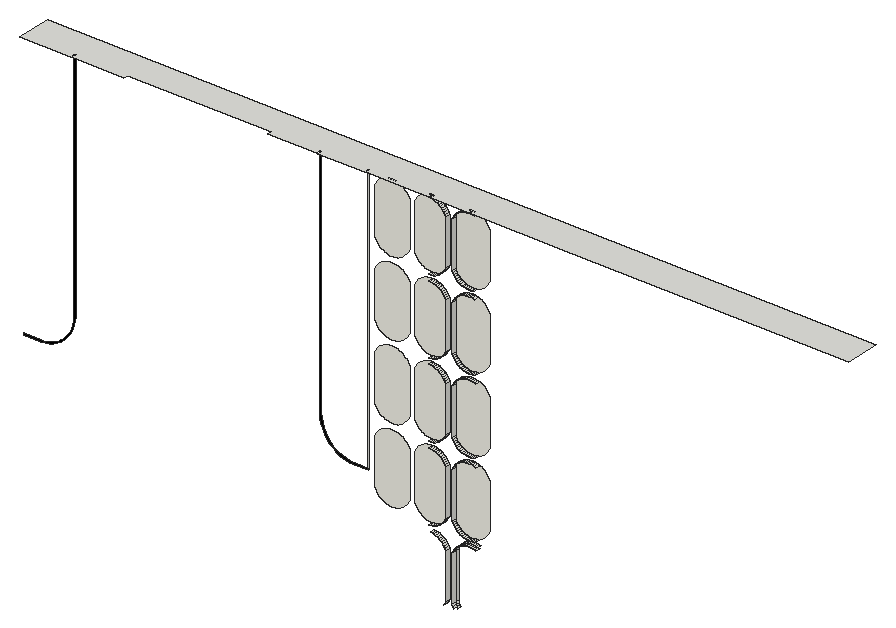
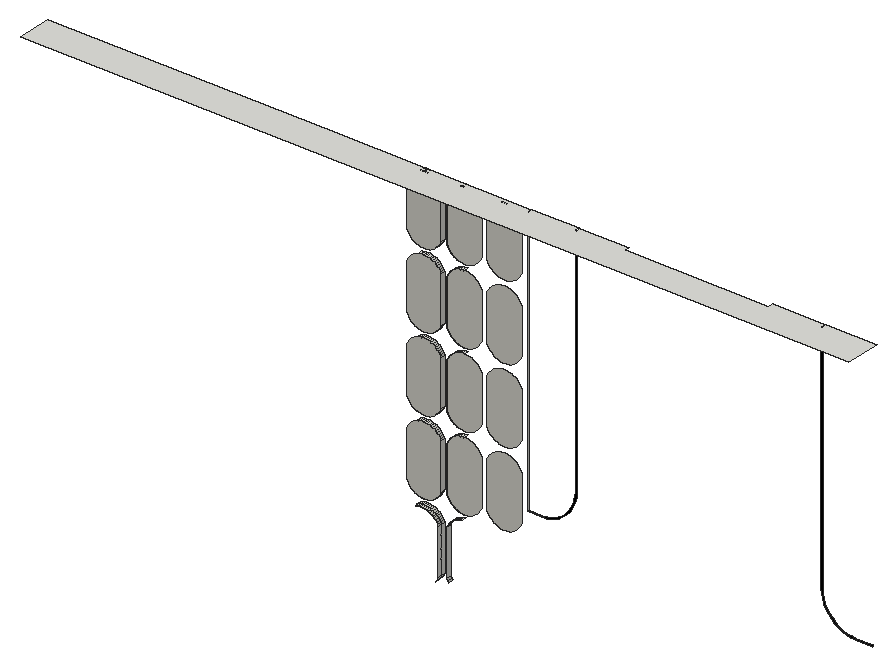
# SketchUp Ruby script. Lengths in inches.
U = 1.inch
M = Sketchup.active_model
def pt(a) = Geom::Point3d.new(a.map { |v| v * U })
def face(e, loops, mat)
  f = e.add_face(loops[0].map { |a| pt(a) })
  loops[1..].each { |l| e.add_face(l.map { |a| pt(a) }).erase! }
  f.material = f.back_material = mat if mat
  f
end
# faces: each face lists its corners as indices into pts; further lists are holes
def faces(e, pts, list, mat = nil) = list.each { |f| face(e, (f[0].is_a?(Array) ? f : [f]).map { |l| l.map { |i| pts[i] } }, mat) }
# xy, xz, yz: faces in a plane at the given z, y or x. An outline is a flat list of corners, or four numbers for a rectangle; further outlines are holes
def ring(l) = l.size == 4 ? [[l[0], l[1]], [l[2], l[1]], [l[2], l[3]], [l[0], l[3]]] : l.each_slice(2).to_a
def flat(e, list, mat, &to3) = list.each { |f| face(e, (f[0].is_a?(Array) ? f : [f]).map { |l| ring(l).map { |u, v| to3.(u, v) } }, mat) }
def xy(e, z, list, mat = nil) = flat(e, list, mat) { |x, y| [x, y, z] }
def xz(e, y, list, mat = nil) = flat(e, list, mat) { |x, z| [x, y, z] }
def yz(e, x, list, mat = nil) = flat(e, list, mat) { |y, z| [x, y, z] }
def lines(e, pts, list) = list.each { |a, b| e.add_line(pt(pts[a]), pt(pts[b])) }
# prism: a flat outline (further loops are holes) pulled along v
def prism(e, loops, v, mat = nil)
  f = face(e, loops, mat); d = Geom::Vector3d.new(v.map { |x| x * U })
  f.pushpull(f.normal.samedirection?(d) ? d.length : -d.length)
end
def box(e, o, s, mat = nil) = prism(e, [[o, [o[0] + s[0], o[1], o[2]], [o[0] + s[0], o[1] + s[1], o[2]], [o[0], o[1] + s[1], o[2]]]], [0, 0, s[2]], mat)
def at(x, y, z, deg = 0) = Geom::Transformation.translation(pt([x, y, z])) * Geom::Transformation.rotation(ORIGIN, Z_AXIS, deg.degrees)
def axes(o, x, y, z) = Geom::Transformation.new([*x, 0, *y, 0, *z, 0, *pt(o).to_a, 1])
def part(name) = M.definitions.add(name)
# library, detail: a bought-in or finely detailed component or shape, given as its bounding box
def library(name, o, s) = part(name).tap { |d| box(d.entities, o, s) }
def detail(e, o, s) = box(e.add_group.entities, o, s)
def put(e, d, t, mat = nil) = e.add_instance(d, t).tap { |i| i.material = mat if mat }
def group(e, t, mat = nil) = e.add_group.tap { |g| g.transformation = t; g.material = mat if mat }.entities
root = M.entities
M.materials.add("Tafisa-Gardenia-or-Gardenia-PM775-4K").color = [246, 245, 235]
M.materials.add("[Color M09]").color = [0, 0, 0]
xy(root,114,[[4.5,138,13.26,138,13.26,138.71,13.5,138.71,13.5,138,22.5,138,22.5,138.79,47.5,138.79,47.5,138,56,138,56,138.71,56.24,138.71,56.24,138,64.38,138,64.38,138.71,64.5,138.71,64.5,138,100.5,138,100.5,138.71,100.62,138.71,100.62,138,148.5,138,148.5,144,4.5,144]])
xz(root,138.71,[[64.38,67.55,64.5,114]])
xz(root,138.71,[[4.5,67.3125,7.5,67.3125,8.28,67.36,9.05,67.52,9.8,67.77,10.5,68.12,11.15,68.55,11.74,69.07,12.26,69.66,12.7,70.3125,13.04,71.02,13.3,71.76,13.45,72.53,13.5,73.3125,13.5,114,13.26,114,13.26,73.3125,13.21,72.56,13.07,71.82,12.83,71.11,12.49,70.43,12.07,69.8,11.58,69.24,11.01,68.74,10.38,68.32,9.71,67.99,8.99,67.75,8.25,67.6,7.5,67.55,4.5,67.55],[62,67.3125,64.5,67.3125,64.5,67.55,62,67.55,61.25,67.6,60.51,67.75,59.79,67.99,59.12,68.32,58.49,68.74,57.92,69.24,57.43,69.8,57.01,70.43,56.67,71.11,56.43,71.82,56.29,72.56,56.24,73.3125,56.24,114,56,114,56,73.3125,56.05,72.53,56.2,71.76,56.46,71.02,56.8,70.3125,57.24,69.66,57.76,69.07,58.35,68.55,59,68.12,59.7,67.77,60.45,67.52,61.22,67.36]],"[Color M09]")
xz(root,138.79,[[68.5,63,68.82,63.02,69.13,63.0625,69.44,63.14,69.74,63.25,70.03,63.38,70.3,63.55,70.56,63.74,70.79,63.95,71.01,64.18,71.2,64.44,71.36,64.71,71.5,65,71.5,73,71.36,73.29,71.2,73.56,71.01,73.82,70.79,74.05,70.56,74.26,70.3,74.45,70.03,74.62,69.74,74.75,69.44,74.86,69.13,74.9375,68.82,74.98,68.5,75,68.18,74.98,67.87,74.9375,67.56,74.86,67.26,74.75,66.97,74.62,66.7,74.45,66.44,74.26,66.21,74.05,65.99,73.82,65.8,73.56,65.64,73.29,65.5,73,65.5,65,65.64,64.71,65.8,64.44,65.99,64.18,66.21,63.95,66.44,63.74,66.7,63.55,66.97,63.38,67.26,63.25,67.56,63.14,67.87,63.0625,68.18,63.02],[75.5,63,75.82,63.02,76.13,63.0625,76.44,63.14,76.74,63.25,77.03,63.38,77.3,63.55,77.56,63.74,77.79,63.95,78.01,64.18,78.2,64.44,78.36,64.71,78.5,65,78.5,73,78.36,73.29,78.2,73.56,78.01,73.82,77.79,74.05,77.56,74.26,77.3,74.45,77.03,74.62,76.74,74.75,76.44,74.86,76.13,74.9375,75.82,74.98,75.5,75,75.18,74.98,74.87,74.9375,74.56,74.86,74.26,74.75,73.97,74.62,73.7,74.45,73.44,74.26,73.21,74.05,72.99,73.82,72.8,73.56,72.64,73.29,72.5,73,72.5,65,72.64,64.71,72.8,64.44,72.99,64.18,73.21,63.95,73.44,63.74,73.7,63.55,73.97,63.38,74.26,63.25,74.56,63.14,74.87,63.0625,75.18,63.02],[82.5,63,82.82,63.02,83.13,63.0625,83.44,63.14,83.74,63.25,84.03,63.38,84.3,63.55,84.56,63.74,84.79,63.95,85.01,64.18,85.2,64.44,85.36,64.71,85.5,65,85.5,73,85.36,73.29,85.2,73.56,85.01,73.82,84.79,74.05,84.56,74.26,84.3,74.45,84.03,74.62,83.74,74.75,83.44,74.86,83.13,74.9375,82.82,74.98,82.5,75,82.18,74.98,81.87,74.9375,81.56,74.86,81.26,74.75,80.97,74.62,80.7,74.45,80.44,74.26,80.21,74.05,79.99,73.82,79.8,73.56,79.64,73.29,79.5,73,79.5,65,79.64,64.71,79.8,64.44,79.99,64.18,80.21,63.95,80.44,63.74,80.7,63.55,80.97,63.38,81.26,63.25,81.56,63.14,81.87,63.0625,82.18,63.02],[68.5,76,68.82,76.02,69.13,76.0625,69.44,76.14,69.74,76.25,70.03,76.38,70.3,76.55,70.56,76.74,70.79,76.95,71.01,77.18,71.2,77.44,71.36,77.71,71.5,78,71.5,86,71.36,86.29,71.2,86.56,71.01,86.82,70.79,87.05,70.56,87.26,70.3,87.45,70.03,87.62,69.74,87.75,69.44,87.86,69.13,87.9375,68.82,87.98,68.5,88,68.18,87.98,67.87,87.9375,67.56,87.86,67.26,87.75,66.97,87.62,66.7,87.45,66.44,87.26,66.21,87.05,65.99,86.82,65.8,86.56,65.64,86.29,65.5,86,65.5,78,65.64,77.71,65.8,77.44,65.99,77.18,66.21,76.95,66.44,76.74,66.7,76.55,66.97,76.38,67.26,76.25,67.56,76.14,67.87,76.0625,68.18,76.02],[75.5,76,75.82,76.02,76.13,76.0625,76.44,76.14,76.74,76.25,77.03,76.38,77.3,76.55,77.56,76.74,77.79,76.95,78.01,77.18,78.2,77.44,78.36,77.71,78.5,78,78.5,86,78.36,86.29,78.2,86.56,78.01,86.82,77.79,87.05,77.56,87.26,77.3,87.45,77.03,87.62,76.74,87.75,76.44,87.86,76.13,87.9375,75.82,87.98,75.5,88,75.18,87.98,74.87,87.9375,74.56,87.86,74.26,87.75,73.97,87.62,73.7,87.45,73.44,87.26,73.21,87.05,72.99,86.82,72.8,86.56,72.64,86.29,72.5,86,72.5,78,72.64,77.71,72.8,77.44,72.99,77.18,73.21,76.95,73.44,76.74,73.7,76.55,73.97,76.38,74.26,76.25,74.56,76.14,74.87,76.0625,75.18,76.02],
  [82.5,76,82.82,76.02,83.13,76.0625,83.44,76.14,83.74,76.25,84.03,76.38,84.3,76.55,84.56,76.74,84.79,76.95,85.01,77.18,85.2,77.44,85.36,77.71,85.5,78,85.5,86,85.36,86.29,85.2,86.56,85.01,86.82,84.79,87.05,84.56,87.26,84.3,87.45,84.03,87.62,83.74,87.75,83.44,87.86,83.13,87.9375,82.82,87.98,82.5,88,82.18,87.98,81.87,87.9375,81.56,87.86,81.26,87.75,80.97,87.62,80.7,87.45,80.44,87.26,80.21,87.05,79.99,86.82,79.8,86.56,79.64,86.29,79.5,86,79.5,78,79.64,77.71,79.8,77.44,79.99,77.18,80.21,76.95,80.44,76.74,80.7,76.55,80.97,76.38,81.26,76.25,81.56,76.14,81.87,76.0625,82.18,76.02],[68.5,89,68.82,89.02,69.13,89.0625,69.44,89.14,69.74,89.25,70.03,89.38,70.3,89.55,70.56,89.74,70.79,89.95,71.01,90.18,71.2,90.44,71.36,90.71,71.5,91,71.5,99,71.36,99.29,71.2,99.56,71.01,99.82,70.79,100.05,70.56,100.26,70.3,100.45,70.03,100.62,69.74,100.75,69.44,100.86,69.13,100.9375,68.82,100.98,68.5,101,68.18,100.98,67.87,100.9375,67.56,100.86,67.26,100.75,66.97,100.62,66.7,100.45,66.44,100.26,66.21,100.05,65.99,99.82,65.8,99.56,65.64,99.29,65.5,99,65.5,91,65.64,90.71,65.8,90.44,65.99,90.18,66.21,89.95,66.44,89.74,66.7,89.55,66.97,89.38,67.26,89.25,67.56,89.14,67.87,89.0625,68.18,89.02],[75.5,89,75.82,89.02,76.13,89.0625,76.44,89.14,76.74,89.25,77.03,89.38,77.3,89.55,77.56,89.74,77.79,89.95,78.01,90.18,78.2,90.44,78.36,90.71,78.5,91,78.5,99,78.36,99.29,78.2,99.56,78.01,99.82,77.79,100.05,77.56,100.26,77.3,100.45,77.03,100.62,76.74,100.75,76.44,100.86,76.13,100.9375,75.82,100.98,75.5,101,75.18,100.98,74.87,100.9375,74.56,100.86,74.26,100.75,73.97,100.62,73.7,100.45,73.44,100.26,73.21,100.05,72.99,99.82,72.8,99.56,72.64,99.29,72.5,99,72.5,91,72.64,90.71,72.8,90.44,72.99,90.18,73.21,89.95,73.44,89.74,73.7,89.55,73.97,89.38,74.26,89.25,74.56,89.14,74.87,89.0625,75.18,89.02],[82.5,89,82.82,89.02,83.13,89.0625,83.44,89.14,83.74,89.25,84.03,89.38,84.3,89.55,84.56,89.74,84.79,89.95,85.01,90.18,85.2,90.44,85.36,90.71,85.5,91,85.5,99,85.36,99.29,85.2,99.56,85.01,99.82,84.79,100.05,84.56,100.26,84.3,100.45,84.03,100.62,83.74,100.75,83.44,100.86,83.13,100.9375,82.82,100.98,82.5,101,82.18,100.98,81.87,100.9375,81.56,100.86,81.26,100.75,80.97,100.62,80.7,100.45,80.44,100.26,80.21,100.05,79.99,99.82,79.8,99.56,79.64,99.29,79.5,99,79.5,91,79.64,90.71,79.8,90.44,79.99,90.18,80.21,89.95,80.44,89.74,80.7,89.55,80.97,89.38,81.26,89.25,81.56,89.14,81.87,89.0625,82.18,89.02],[68.5,102,68.82,102.02,69.13,102.0625,69.44,102.14,69.74,102.25,70.03,102.38,70.3,102.55,70.56,102.74,70.79,102.95,71.01,103.18,71.2,103.44,71.36,103.71,71.5,104,71.5,112,71.36,112.29,71.2,112.56,71.01,112.82,70.79,113.05,70.56,113.26,70.3,113.45,70.03,113.62,69.74,113.75,69.44,113.86,69.13,113.9375,68.82,113.98,68.5,114,68.18,113.98,67.87,113.9375,67.56,113.86,67.26,113.75,66.97,113.62,66.7,113.45,66.44,113.26,66.21,113.05,65.99,112.82,65.8,112.56,65.64,112.29,65.5,112,65.5,104,65.64,103.71,65.8,103.44,65.99,103.18,66.21,102.95,66.44,102.74,66.7,102.55,66.97,102.38,67.26,102.25,67.56,102.14,67.87,102.0625,68.18,102.02],
  [75.5,102,75.82,102.02,76.13,102.0625,76.44,102.14,76.74,102.25,77.03,102.38,77.3,102.55,77.56,102.74,77.79,102.95,78.01,103.18,78.2,103.44,78.36,103.71,78.5,104,78.5,112,78.36,112.29,78.2,112.56,78.01,112.82,77.79,113.05,77.56,113.26,77.3,113.45,77.03,113.62,76.74,113.75,76.44,113.86,76.13,113.9375,75.82,113.98,75.5,114,75.18,113.98,74.87,113.9375,74.56,113.86,74.26,113.75,73.97,113.62,73.7,113.45,73.44,113.26,73.21,113.05,72.99,112.82,72.8,112.56,72.64,112.29,72.5,112,72.5,104,72.64,103.71,72.8,103.44,72.99,103.18,73.21,102.95,73.44,102.74,73.7,102.55,73.97,102.38,74.26,102.25,74.56,102.14,74.87,102.0625,75.18,102.02],[82.5,102,82.82,102.02,83.13,102.0625,83.44,102.14,83.74,102.25,84.03,102.38,84.3,102.55,84.56,102.74,84.79,102.95,85.01,103.18,85.2,103.44,85.36,103.71,85.5,104,85.5,112,85.36,112.29,85.2,112.56,85.01,112.82,84.79,113.05,84.56,113.26,84.3,113.45,84.03,113.62,83.74,113.75,83.44,113.86,83.13,113.9375,82.82,113.98,82.5,114,82.18,113.98,81.87,113.9375,81.56,113.86,81.26,113.75,80.97,113.62,80.7,113.45,80.44,113.26,80.21,113.05,79.99,112.82,79.8,112.56,79.64,112.29,79.5,112,79.5,104,79.64,103.71,79.8,103.44,79.99,103.18,80.21,102.95,80.44,102.74,80.7,102.55,80.97,102.38,81.26,102.25,81.56,102.14,81.87,102.0625,82.18,102.02]],"Tafisa-Gardenia-or-Gardenia-PM775-4K")
yz(root,78.5,[[138,52,138.79,60],[138,65,138.79,73],[138,78,138.79,86],[138,91,138.79,99],[138,104,138.79,112]])
yz(root,79.5,[[138,52,138.79,60],[138.79,52,139.4375,60],[138,65,138.79,73],[138,78,138.79,86],[138,91,138.79,99],
  [138,104,138.79,112]])
p = [[79.8,139.4375,51.44],[79.8,138.79,51.44],[79.99,138.79,51.18],[79.99,139.4375,51.18],[78.36,138.79,51.71],[78.2,138.79,51.44],
  [78.2,138,51.44],[78.36,138,51.71],[79.64,138.79,51.71],[79.64,138,51.71],[79.8,138,51.44],[79.64,139.4375,51.71],
  [78.5,138.79,52],[78.5,138,52],[79.5,138.79,52],[79.5,138,52],[79.5,139.4375,52],[78.36,138.79,60.29],
  [78.5,138.79,60],[78.5,138,60],[78.36,138,60.29],[79.5,138.79,60],[79.64,138.79,60.29],[79.64,138,60.29],
  [79.5,138,60],[79.64,139.4375,60.29],[79.5,139.4375,60],[78.2,138.79,60.56],[78.2,138,60.56],[79.8,138.79,60.56],
  [79.8,138,60.56],[79.8,139.4375,60.56],[78.01,138.79,60.82],[78.01,138,60.82],[79.99,138.79,60.82],[79.99,138,60.82],
  [79.99,139.4375,60.82],[77.79,138.79,61.05],[77.79,138,61.05],[80.21,138.79,61.05],[80.21,138,61.05],[80.21,139.4375,61.05],
  [77.56,138.79,61.26],[77.56,138,61.26],[80.44,138.79,61.26],[80.44,138,61.26],[80.44,139.4375,61.26],[77.3,138.79,61.45],
  [77.3,138,61.45],[80.7,138.79,61.45],[80.7,138,61.45],[80.7,139.4375,61.45],[77.03,138.79,61.62],[77.03,138,61.62],
  [80.97,138.79,61.62],[80.97,138,61.62],[80.97,139.4375,61.62],[76.74,138.79,61.75],[76.74,138,61.75],[81.26,138.79,61.75],
  [81.26,138,61.75],[81.26,139.4375,61.75],[76.44,138.79,61.86],[76.44,138,61.86],[81.56,138.79,61.86],[81.56,138,61.86],
  [83.44,138.79,61.86],[83.74,138.79,61.75],[83.74,138,61.75],[83.44,138,61.86],[81.56,139.4375,61.86],[75.82,138.79,61.98],
  [76.13,138.79,61.9375],[76.13,138,61.9375],[75.82,138,61.98],[81.87,138.79,61.9375],[81.87,138,61.9375],[82.18,138.79,61.98],
  [82.18,138,61.98],[82.82,138.79,61.98],[83.13,138.79,61.9375],[83.13,138,61.9375],[82.82,138,61.98],[81.87,139.4375,61.9375],
  [82.18,139.4375,61.98],[83.13,139.4375,61.9375],[82.82,139.4375,61.98],[83.44,139.4375,61.86],[82.5,138.79,62],[82.5,138,62],
  [82.5,139.4375,62],[75.82,138.79,63.02],[75.5,138.79,63],[75.5,138,63],[75.82,138,63.02],[76.13,138.79,63.0625],
  [76.13,138,63.0625],[82.18,138.79,63.02],[81.87,138.79,63.0625],[81.87,138,63.0625],[82.18,138,63.02],[82.5,138.79,63],
  [82.5,138,63],[82.82,138.79,63.02],[82.82,138,63.02],[83.13,138.79,63.0625],[83.13,138,63.0625],[76.44,138.79,63.14],
  [76.44,138,63.14],[76.74,138.79,63.25],[76.74,138,63.25],[81.56,138.79,63.14],[81.26,138.79,63.25],[81.26,138,63.25],
  [81.56,138,63.14],[83.44,138.79,63.14],[83.44,138,63.14],[83.74,138.79,63.25],[83.74,138,63.25],[77.03,138.79,63.38],
  [77.03,138,63.38],[80.97,138.79,63.38],[80.97,138,63.38],[77.3,138.79,63.55],[77.3,138,63.55],[80.7,138.79,63.55],
  [80.7,138,63.55],[77.56,138.79,63.74],[77.56,138,63.74],[80.44,138.79,63.74],[80.44,138,63.74],[77.79,138.79,63.95],
  [77.79,138,63.95],[80.21,138.79,63.95],[80.21,138,63.95],[78.01,138.79,64.18],[78.01,138,64.18],[79.99,138.79,64.18],
  [79.99,138,64.18],[78.2,138.79,64.44],[78.2,138,64.44],[79.8,138.79,64.44],[79.8,138,64.44],[78.36,138.79,64.71],
  [78.36,138,64.71],[79.64,138.79,64.71],[79.64,138,64.71],[78.5,138.79,65],[78.5,138,65],[79.5,138.79,65],
  [79.5,138,65],[78.36,138.79,73.29],[78.5,138.79,73],[78.5,138,73],[78.36,138,73.29],[79.5,138.79,73],
  [79.64,138.79,73.29],[79.64,138,73.29],[79.5,138,73],[78.2,138.79,73.56],[78.2,138,73.56],[79.8,138.79,73.56],
  [79.8,138,73.56],[78.01,138.79,73.82],[78.01,138,73.82],[79.99,138.79,73.82],[79.99,138,73.82],[77.79,138.79,74.05],
  [77.79,138,74.05],[80.21,138.79,74.05],[80.21,138,74.05],[77.56,138.79,74.26],[77.56,138,74.26],[80.44,138.79,74.26],
  [80.44,138,74.26],[77.3,138.79,74.45],[77.3,138,74.45],[80.7,138.79,74.45],[80.7,138,74.45],[77.03,138.79,74.62],
  [77.03,138,74.62],[80.97,138.79,74.62],[80.97,138,74.62],[76.74,138.79,74.75],[76.74,138,74.75],[81.26,138.79,74.75],
  [81.26,138,74.75],[76.44,138.79,74.86],[76.44,138,74.86],[81.56,138.79,74.86],[81.56,138,74.86],[83.44,138.79,74.86],
  [83.74,138.79,74.75],[83.74,138,74.75],[83.44,138,74.86],[75.82,138.79,74.98],[76.13,138.79,74.9375],[76.13,138,74.9375],
  [75.82,138,74.98],[81.87,138.79,74.9375],[81.87,138,74.9375],[82.18,138.79,74.98],[82.18,138,74.98],[82.82,138.79,74.98],
  [83.13,138.79,74.9375],[83.13,138,74.9375],[82.82,138,74.98],[75.5,138.79,75],[75.5,138,75],[82.5,138.79,75],
  [82.5,138,75],[75.82,138.79,76.02],[75.5,138.79,76],[75.5,138,76],[75.82,138,76.02],[76.13,138.79,76.0625],
  [76.13,138,76.0625],[82.18,138.79,76.02],[81.87,138.79,76.0625],[81.87,138,76.0625],[82.18,138,76.02],[82.5,138.79,76],
  [82.5,138,76],[82.82,138.79,76.02],[82.82,138,76.02],[83.13,138.79,76.0625],[83.13,138,76.0625],[76.44,138.79,76.14],
  [76.44,138,76.14],[76.74,138.79,76.25],[76.74,138,76.25],[81.56,138.79,76.14],[81.26,138.79,76.25],[81.26,138,76.25],
  [81.56,138,76.14],[83.44,138.79,76.14],[83.44,138,76.14],[83.74,138.79,76.25],[83.74,138,76.25],[77.03,138.79,76.38],
  [77.03,138,76.38],[80.97,138.79,76.38],[80.97,138,76.38],[77.3,138.79,76.55],[77.3,138,76.55],[80.7,138.79,76.55],
  [80.7,138,76.55],[77.56,138.79,76.74],[77.56,138,76.74],[80.44,138.79,76.74],[80.44,138,76.74],[77.79,138.79,76.95],
  [77.79,138,76.95],[80.21,138.79,76.95],[80.21,138,76.95],[78.01,138.79,77.18],[78.01,138,77.18],[79.99,138.79,77.18],
  [79.99,138,77.18],[78.2,138.79,77.44],[78.2,138,77.44],[79.8,138.79,77.44],[79.8,138,77.44],[78.36,138.79,77.71],
  [78.36,138,77.71],[79.64,138.79,77.71],[79.64,138,77.71],[78.5,138.79,78],[78.5,138,78],[79.5,138.79,78],
  [79.5,138,78],[78.36,138.79,86.29],[78.5,138.79,86],[78.5,138,86],[78.36,138,86.29],[79.5,138.79,86],
  [79.64,138.79,86.29],[79.64,138,86.29],[79.5,138,86],[78.2,138.79,86.56],[78.2,138,86.56],[79.8,138.79,86.56],
  [79.8,138,86.56],[78.01,138.79,86.82],[78.01,138,86.82],[79.99,138.79,86.82],[79.99,138,86.82],[77.79,138.79,87.05],
  [77.79,138,87.05],[80.21,138.79,87.05],[80.21,138,87.05],[77.56,138.79,87.26],[77.56,138,87.26],[80.44,138.79,87.26],
  [80.44,138,87.26],[77.3,138.79,87.45],[77.3,138,87.45],[80.7,138.79,87.45],[80.7,138,87.45],[77.03,138.79,87.62],
  [77.03,138,87.62],[80.97,138.79,87.62],[80.97,138,87.62],[76.74,138.79,87.75],[76.74,138,87.75],[81.26,138.79,87.75],
  [81.26,138,87.75],[76.44,138.79,87.86],[76.44,138,87.86],[81.56,138.79,87.86],[81.56,138,87.86],[83.44,138.79,87.86],
  [83.74,138.79,87.75],[83.74,138,87.75],[83.44,138,87.86],[75.82,138.79,87.98],[76.13,138.79,87.9375],[76.13,138,87.9375],
  [75.82,138,87.98],[81.87,138.79,87.9375],[81.87,138,87.9375],[82.18,138.79,87.98],[82.18,138,87.98],[82.82,138.79,87.98],
  [83.13,138.79,87.9375],[83.13,138,87.9375],[82.82,138,87.98],[75.5,138.79,88],[75.5,138,88],[82.5,138.79,88],
  [82.5,138,88],[75.82,138.79,89.02],[75.5,138.79,89],[75.5,138,89],[75.82,138,89.02],[76.13,138.79,89.0625],
  [76.13,138,89.0625],[82.18,138.79,89.02],[81.87,138.79,89.0625],[81.87,138,89.0625],[82.18,138,89.02],[82.5,138.79,89],
  [82.5,138,89],[82.82,138.79,89.02],[82.82,138,89.02],[83.13,138.79,89.0625],[83.13,138,89.0625],[76.44,138.79,89.14],
  [76.44,138,89.14],[76.74,138.79,89.25],[76.74,138,89.25],[81.56,138.79,89.14],[81.26,138.79,89.25],[81.26,138,89.25],
  [81.56,138,89.14],[83.44,138.79,89.14],[83.44,138,89.14],[83.74,138.79,89.25],[83.74,138,89.25],[77.03,138.79,89.38],
  [77.03,138,89.38],[80.97,138.79,89.38],[80.97,138,89.38],[77.3,138.79,89.55],[77.3,138,89.55],[80.7,138.79,89.55],
  [80.7,138,89.55],[77.56,138.79,89.74],[77.56,138,89.74],[80.44,138.79,89.74],[80.44,138,89.74],[77.79,138.79,89.95],
  [77.79,138,89.95],[80.21,138.79,89.95],[80.21,138,89.95],[78.01,138.79,90.18],[78.01,138,90.18],[79.99,138.79,90.18],
  [79.99,138,90.18],[78.2,138.79,90.44],[78.2,138,90.44],[79.8,138.79,90.44],[79.8,138,90.44],[78.36,138.79,90.71],
  [78.36,138,90.71],[79.64,138.79,90.71],[79.64,138,90.71],[78.5,138.79,91],[78.5,138,91],[79.5,138.79,91],
  [79.5,138,91],[78.36,138.79,99.29],[78.5,138.79,99],[78.5,138,99],[78.36,138,99.29],[79.5,138.79,99],
  [79.64,138.79,99.29],[79.64,138,99.29],[79.5,138,99],[78.2,138.79,99.56],[78.2,138,99.56],[79.8,138.79,99.56],
  [79.8,138,99.56],[78.01,138.79,99.82],[78.01,138,99.82],[79.99,138.79,99.82],[79.99,138,99.82],[77.79,138.79,100.05],
  [77.79,138,100.05],[80.21,138.79,100.05],[80.21,138,100.05],[77.56,138.79,100.26],[77.56,138,100.26],[80.44,138.79,100.26],
  [80.44,138,100.26],[77.3,138.79,100.45],[77.3,138,100.45],[80.7,138.79,100.45],[80.7,138,100.45],[77.03,138.79,100.62],
  [77.03,138,100.62],[80.97,138.79,100.62],[80.97,138,100.62],[76.74,138.79,100.75],[76.74,138,100.75],[81.26,138.79,100.75],
  [81.26,138,100.75],[76.44,138.79,100.86],[76.44,138,100.86],[81.56,138.79,100.86],[81.56,138,100.86],[75.82,138.79,100.98],
  [76.13,138.79,100.9375],[76.13,138,100.9375],[75.82,138,100.98],[81.87,138.79,100.9375],[81.87,138,100.9375],[82.18,138.79,100.98],
  [82.18,138,100.98],[82.82,138.79,100.98],[83.13,138.79,100.9375],[83.13,138,100.9375],[82.82,138,100.98],[83.44,138.79,100.86],
  [83.44,138,100.86],[75.5,138.79,101],[75.5,138,101],[82.5,138.79,101],[82.5,138,101],[75.82,138.79,102.02],
  [75.5,138.79,102],[75.5,138,102],[75.82,138,102.02],[76.13,138.79,102.0625],[76.13,138,102.0625],[82.18,138.79,102.02],
  [81.87,138.79,102.0625],[81.87,138,102.0625],[82.18,138,102.02],[82.5,138.79,102],[82.5,138,102],[82.82,138.79,102.02],
  [82.82,138,102.02],[83.13,138.79,102.0625],[83.13,138,102.0625],[76.44,138.79,102.14],[76.44,138,102.14],[76.74,138.79,102.25],
  [76.74,138,102.25],[81.56,138.79,102.14],[81.26,138.79,102.25],[81.26,138,102.25],[81.56,138,102.14],[83.44,138.79,102.14],
  [83.44,138,102.14],[77.03,138.79,102.38],[77.03,138,102.38],[80.97,138.79,102.38],[80.97,138,102.38],[77.3,138.79,102.55],
  [77.3,138,102.55],[80.7,138.79,102.55],[80.7,138,102.55],[77.56,138.79,102.74],[77.56,138,102.74],[80.44,138.79,102.74],
  [80.44,138,102.74],[77.79,138.79,102.95],[77.79,138,102.95],[80.21,138.79,102.95],[80.21,138,102.95],[78.01,138.79,103.18],
  [78.01,138,103.18],[79.99,138.79,103.18],[79.99,138,103.18],[78.2,138.79,103.44],[78.2,138,103.44],[79.8,138.79,103.44],
  [79.8,138,103.44],[78.36,138.79,103.71],[78.36,138,103.71],[79.64,138.79,103.71],[79.64,138,103.71],[78.5,138.79,104],
  [78.5,138,104],[79.5,138.79,104],[79.5,138,104],[78.36,138.79,112.29],[78.5,138.79,112],[78.5,138,112],
  [78.36,138,112.29],[79.5,138.79,112],[79.64,138.79,112.29],[79.64,138,112.29],[79.5,138,112],[78.2,138.79,112.56],
  [78.2,138,112.56],[79.8,138.79,112.56],[79.8,138,112.56],[78.01,138.79,112.82],[78.01,138,112.82],[79.99,138.79,112.82],
  [79.99,138,112.82],[77.79,138.79,113.05],[77.79,138,113.05],[80.21,138.79,113.05],[80.21,138,113.05],[77.56,138.79,113.26],
  [77.56,138,113.26],[80.44,138.79,113.26],[80.44,138,113.26],[77.3,138.79,113.45],[77.3,138,113.45],[80.7,138.79,113.45],
  [80.7,138,113.45],[77.03,138.79,113.62],[77.03,138,113.62],[80.97,138.79,113.62],[80.97,138,113.62],[76.74,138.79,113.75],
  [76.74,138,113.75],[81.26,138.79,113.75],[81.26,138,113.75],[76.44,138.79,113.86],[76.44,138,113.86],[81.56,138.79,113.86],
  [81.56,138,113.86],[75.82,138.79,113.98],[76.13,138.79,113.9375],[76.13,138,113.9375],[75.82,138,113.98],[81.87,138.79,113.9375],
  [81.87,138,113.9375],[82.18,138.79,113.98],[82.18,138,113.98],[82.82,138.79,113.98],[83.13,138.79,113.9375],[83.13,138,113.9375],
  [82.82,138,113.98],[83.44,138.79,113.86],[83.44,138,113.86],[75.5,138.79,114],[75.5,138,114],[82.5,138.79,114],
  [82.5,138,114]]
faces(root,p,[[0,1,2,3],[4,5,6,7],[1,8,9,10],[11,8,1,0],[12,4,7,13],[8,14,15,9],[16,14,8,11],[17,18,19,20],
  [21,22,23,24],[25,22,21,26],[27,17,20,28],[22,29,30,23],[31,29,22,25],[32,27,28,33],[29,34,35,30],[36,34,29,31],
  [37,32,33,38],[34,39,40,35],[41,39,34,36],[42,37,38,43],[39,44,45,40],[46,44,39,41],[47,42,43,48],[44,49,50,45],
  [51,49,44,46],[52,47,48,53],[49,54,55,50],[56,54,49,51],[57,52,53,58],[54,59,60,55],[61,59,54,56],[62,57,58,63],
  [59,64,65,60],[66,67,68,69],[70,64,59,61],[71,72,73,74],[72,62,63,73],[64,75,76,65],[75,77,78,76],[79,80,81,82],
  [80,66,69,81],[83,75,64,70],[84,77,75,83],[85,80,79,86],[87,66,80,85],[77,88,89,78],[88,79,82,89],[90,88,77,84],
  [86,79,88,90],[91,92,93,94],[95,91,94,96],[97,98,99,100],[101,97,100,102],[103,101,102,104],[105,103,104,106],[107,95,96,108],
  [109,107,108,110],[111,112,113,114],[98,111,114,99],[115,105,106,116],[117,115,116,118],[119,109,110,120],[112,121,122,113],[123,119,120,124],
  [121,125,126,122],[127,123,124,128],[125,129,130,126],[131,127,128,132],[129,133,134,130],[135,131,132,136],[133,137,138,134],[139,135,136,140],
  [137,141,142,138],[143,139,140,144],[141,145,146,142],[147,143,144,148],[145,149,150,146],[151,152,153,154],[155,156,157,158],[159,151,154,160],
  [156,161,162,157],[163,159,160,164],[161,165,166,162],[167,163,164,168],[165,169,170,166],[171,167,168,172],[169,173,174,170],[175,171,172,176],
  [173,177,178,174],[179,175,176,180],[177,181,182,178],[183,179,180,184],[181,185,186,182],[187,183,184,188],[185,189,190,186],[191,192,193,194],
  [195,196,197,198],[196,187,188,197],[189,199,200,190],[199,201,202,200],[203,204,205,206],[204,191,194,205],[207,195,198,208],[201,209,210,202],
  [209,203,206,210],[211,212,213,214],[215,211,214,216],[217,218,219,220],[221,217,220,222],[223,221,222,224],[225,223,224,226],[227,215,216,228],
  [229,227,228,230],[231,232,233,234],[218,231,234,219],[235,225,226,236],[237,235,236,238],[239,229,230,240],[232,241,242,233],[243,239,240,244],
  [241,245,246,242],[247,243,244,248],[245,249,250,246],[251,247,248,252],[249,253,254,250],[255,251,252,256],[253,257,258,254],[259,255,256,260],
  [257,261,262,258],[263,259,260,264],[261,265,266,262],[267,263,264,268],[265,269,270,266],[271,272,273,274],[275,276,277,278],[279,271,274,280],
  [276,281,282,277],[283,279,280,284],[281,285,286,282],[287,283,284,288],[285,289,290,286],[291,287,288,292],[289,293,294,290],[295,291,292,296],
  [293,297,298,294],[299,295,296,300],[297,301,302,298],[303,299,300,304],[301,305,306,302],[307,303,304,308],[305,309,310,306],[311,312,313,314],
  [315,316,317,318],[316,307,308,317],[309,319,320,310],[319,321,322,320],[323,324,325,326],[324,311,314,325],[327,315,318,328],[321,329,330,322],
  [329,323,326,330],[331,332,333,334],[335,331,334,336],[337,338,339,340],[341,337,340,342],[343,341,342,344],[345,343,344,346],[347,335,336,348],
  [349,347,348,350],[351,352,353,354],[338,351,354,339],[355,345,346,356],[357,355,356,358],[359,349,350,360],[352,361,362,353],[363,359,360,364],
  [361,365,366,362],[367,363,364,368],[365,369,370,366],[371,367,368,372],[369,373,374,370],[375,371,372,376],[373,377,378,374],[379,375,376,380],
  [377,381,382,378],[383,379,380,384],[381,385,386,382],[387,383,384,388],[385,389,390,386],[391,392,393,394],[395,396,397,398],[399,391,394,400],
  [396,401,402,397],[403,399,400,404],[401,405,406,402],[407,403,404,408],[405,409,410,406],[411,407,408,412],[409,413,414,410],[415,411,412,416],
  [413,417,418,414],[419,415,416,420],[417,421,422,418],[423,419,420,424],[421,425,426,422],[427,423,424,428],[425,429,430,426],[431,432,433,434],
  [432,427,428,433],[429,435,436,430],[435,437,438,436],[439,440,441,442],[440,443,444,441],[445,431,434,446],[437,447,448,438],[447,439,442,448],
  [449,450,451,452],[453,449,452,454],[455,456,457,458],[459,455,458,460],[461,459,460,462],[463,461,462,464],[465,453,454,466],[467,465,466,468],
  [469,470,471,472],[456,469,472,457],[473,463,464,474],[475,467,468,476],[470,477,478,471],[479,475,476,480],[477,481,482,478],[483,479,480,484],
  [481,485,486,482],[487,483,484,488],[485,489,490,486],[491,487,488,492],[489,493,494,490],[495,491,492,496],[493,497,498,494],[499,495,496,500],
  [497,501,502,498],[503,499,500,504],[501,505,506,502],[507,508,509,510],[511,512,513,514],[515,507,510,516],[512,517,518,513],[519,515,516,520],
  [517,521,522,518],[523,519,520,524],[521,525,526,522],[527,523,524,528],[525,529,530,526],[531,527,528,532],[529,533,534,530],[535,531,532,536],
  [533,537,538,534],[539,535,536,540],[537,541,542,538],[543,539,540,544],[541,545,546,542],[547,548,549,550],[548,543,544,549],[545,551,552,546],
  [551,553,554,552],[555,556,557,558],[556,559,560,557],[561,547,550,562],[553,563,564,554],[563,555,558,564]])
